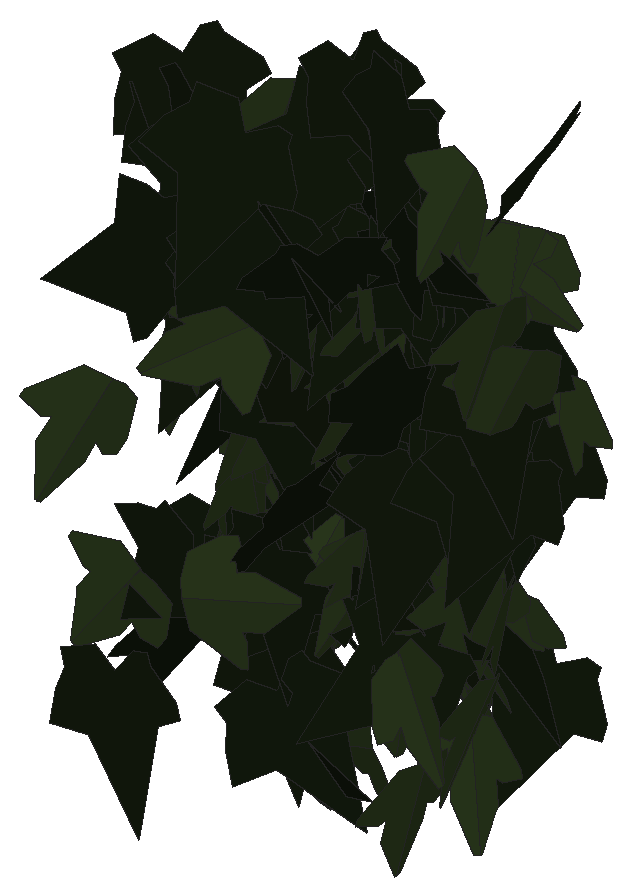
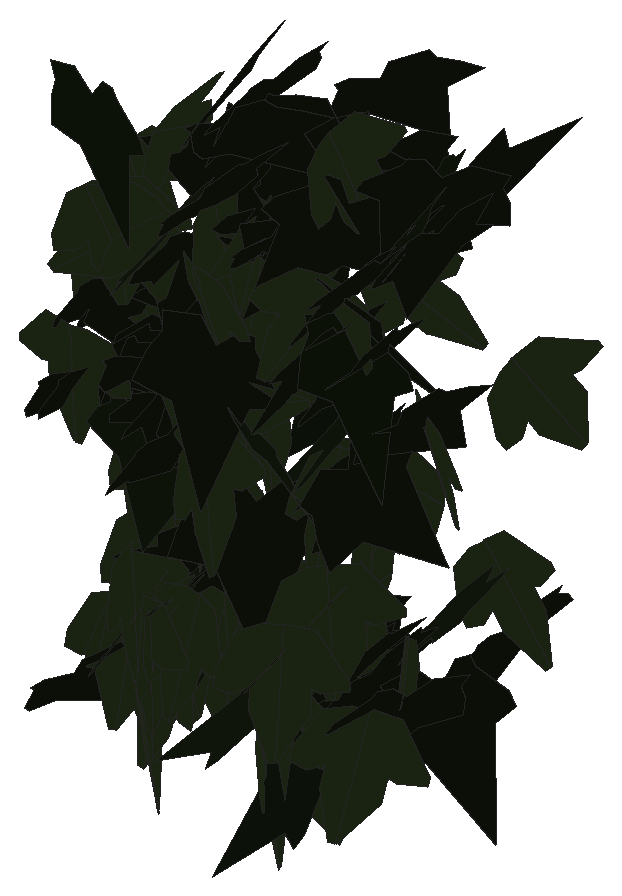
# SketchUp Ruby script. Lengths in inches.
U = 1.inch
M = Sketchup.active_model
def pt(a) = Geom::Point3d.new(a.map { |v| v * U })
def face(e, loops, mat)
  f = e.add_face(loops[0].map { |a| pt(a) })
  loops[1..].each { |l| e.add_face(l.map { |a| pt(a) }).erase! }
  f.material = f.back_material = mat if mat
  f
end
# faces: each face lists its corners as indices into pts; further lists are holes
def faces(e, pts, list, mat = nil) = list.each { |f| face(e, (f[0].is_a?(Array) ? f : [f]).map { |l| l.map { |i| pts[i] } }, mat) }
# xy, xz, yz: faces in a plane at the given z, y or x. An outline is a flat list of corners, or four numbers for a rectangle; further outlines are holes
def ring(l) = l.size == 4 ? [[l[0], l[1]], [l[2], l[1]], [l[2], l[3]], [l[0], l[3]]] : l.each_slice(2).to_a
def flat(e, list, mat, &to3) = list.each { |f| face(e, (f[0].is_a?(Array) ? f : [f]).map { |l| ring(l).map { |u, v| to3.(u, v) } }, mat) }
def xy(e, z, list, mat = nil) = flat(e, list, mat) { |x, y| [x, y, z] }
def xz(e, y, list, mat = nil) = flat(e, list, mat) { |x, z| [x, y, z] }
def yz(e, x, list, mat = nil) = flat(e, list, mat) { |y, z| [x, y, z] }
def lines(e, pts, list) = list.each { |a, b| e.add_line(pt(pts[a]), pt(pts[b])) }
# prism: a flat outline (further loops are holes) pulled along v
def prism(e, loops, v, mat = nil)
  f = face(e, loops, mat); d = Geom::Vector3d.new(v.map { |x| x * U })
  f.pushpull(f.normal.samedirection?(d) ? d.length : -d.length)
end
def box(e, o, s, mat = nil) = prism(e, [[o, [o[0] + s[0], o[1], o[2]], [o[0] + s[0], o[1] + s[1], o[2]], [o[0], o[1] + s[1], o[2]]]], [0, 0, s[2]], mat)
def at(x, y, z, deg = 0) = Geom::Transformation.translation(pt([x, y, z])) * Geom::Transformation.rotation(ORIGIN, Z_AXIS, deg.degrees)
def axes(o, x, y, z) = Geom::Transformation.new([*x, 0, *y, 0, *z, 0, *pt(o).to_a, 1])
def part(name) = M.definitions.add(name)
# library, detail: a bought-in or finely detailed component or shape, given as its bounding box
def library(name, o, s) = part(name).tap { |d| box(d.entities, o, s) }
def detail(e, o, s) = box(e.add_group.entities, o, s)
def put(e, d, t, mat = nil) = e.add_instance(d, t).tap { |i| i.material = mat if mat }
def group(e, t, mat = nil) = e.add_group.tap { |g| g.transformation = t; g.material = mat if mat }.entities
root = M.entities
M.materials.add("efeu1").color = [18, 25, 13]
M.materials.add("efeu2").color = [43, 57, 29]
c1 = part("ivyleaf_10")
p = [[0,0.5,-0.03],[-0.0625,2.02,-0.43],[-0.19,2.01,-0.46],[-0.54,1.05,-0.29],[-0.52,0.625,-0.18],[-0.83,0.76,-0.28],
  [-1.16,0.64,-0.33],[-1.15,0.33,-0.24],[-0.77,-0.39,0.02],[-0.3,-0.51,0.16],[0.04,-0.48,0.23],[-0.02,2.01,-0.4375],
  [-0.06,2.01,-0.43],[0.04,-0.49,0.23],[0.67,-0.49,0.14],[1.38,0.36,-0.2],[1.375,0.51,-0.24],[0.81,0.65,-0.19],
  [0.62,0.59,-0.15],[0.6,1.09,-0.28],[0.5,1.23,-0.31]]
faces(c1.entities,p,[[0,1,2,3,4,5,6,7,8,9,10],[11,12,0,13,14,15,16,17,18,19,20]],"efeu2")
c2 = part("ivyleaf_9")
p = [[1.54,2.16,1.25],[1.36,2.04,1.19],[-0.21,0.99,0.68],[-0.71,1.11,0.82],[-0.85,0.86,0.67],[-0.8,0.17,0.21],
  [-0.9,-0.01,0.1],[-0.67,-0.16,-0.02],[-0.08,-0.08,-0.05],[-0.03,-0.6,-0.4],[0.65,-0.88,-0.66],[0.83,-0.6,-0.49],
  [1.29,-0.42,-0.43],[1.8125,-0.07,-0.26],[1.21,0.44,0.15]]
faces(c2.entities,p,[[0,1,2,3,4,5,6,7,8,9,10,11,12,13,14]],"efeu1")
put(root,c1,axes([30.6875,222.58,242.9],[-0.44057,-0.22233,-0.08041],[0.0674,0.04488,-0.4934],[0.22661,-0.44559,-0.00958]))
put(root,c2,axes([30.85,221.21,242.7],[-0.04956,0.42875,-0.25242],[0.01989,-0.25176,-0.43153],[-0.49714,-0.05281,0.0079]))
put(root,c2,axes([30.53,222.15,243.15],[0.04788,-0.4175,-0.27092],[0.04263,0.27461,-0.41566],[0.49587,0.0167,0.06189]))
put(root,c1,axes([31.03,220.24,243.5],[-0.38302,-0.03283,0.31972],[-0.30495,-0.11998,-0.37764],[0.10152,-0.48428,0.07189]))
put(root,c1,axes([30.85,219.97,245.4],[-0.17761,-0.35591,0.30295],[-0.01741,-0.31883,-0.38477],[0.46707,-0.14722,0.10086]))
put(root,c2,axes([30.625,221.55,247.65],[0.05449,-0.47877,-0.13345],[-0.02033,0.13199,-0.48183],[0.49661,0.05793,-0.00509]))
put(root,c1,axes([30.84,221.72,243.2],[0.20355,-0.37433,-0.26162],[0.0043,0.28799,-0.40871],[0.45667,0.16414,0.12045]))
put(root,c2,axes([30.67,221.46,248.16],[-0.10102,-0.34742,-0.3451],[0.15224,0.31262,-0.35929],[0.46542,-0.17767,0.04262]))
put(root,c1,axes([30.85,221.37,245.48],[0.38535,-0.31856,0.00527],[0.00218,-0.00562,-0.49996],[0.31859,0.38534,-0.00294]))
put(root,c2,axes([30.87,221.78,245.71],[-0.19367,-0.44322,0.12668],[-0.0312,-0.12449,-0.48325],[0.45991,-0.19508,0.02057]))
put(root,c2,axes([30.96,221.17,243.27],[-0.20265,-0.2775,0.36322],[0.04048,-0.40665,-0.28809],[0.4553,-0.08736,0.18728]))
put(root,c2,axes([30.79,221.49,247.84],[0.30364,-0.39724,-0.0029],[-0.00494,-0.00013,-0.49998],[0.39722,0.30365,-0.004]))
put(root,c1,axes([31.23,222.4,244.11],[-0.37027,-0.33239,0.04918],[-0.00503,-0.06769,-0.49537],[0.33597,-0.36733,0.04678]))
put(root,c2,axes([31.12,221.36,247.33],[-0.16184,-0.44057,0.17236],[-0.03359,-0.17101,-0.46864],[0.47189,-0.16327,0.02576]))
put(root,c2,axes([31.28,221.97,245.15],[-0.13045,0.21943,-0.42992],[0.13528,-0.41088,-0.25075],[-0.46334,-0.18174,0.04783]))
put(root,c2,axes([31.39,221.81,246.35],[-0.115,0.48614,-0.02096],[0.00787,-0.01967,-0.49955],[-0.48653,-0.11522,-0.00312]))
put(root,c2,axes([31.1,219.94,242.69],[0.06343,-0.49327,-0.05162],[0.00258,0.05236,-0.49724],[0.49595,0.06282,0.00919]))
put(root,c2,axes([31.04,221.91,247.35],[0.20706,-0.40476,-0.20807],[0.02398,0.23798,-0.43908],[0.45448,0.17186,0.11797]))
put(root,c1,axes([31.4,222.88,243.65],[-0.46203,-0.18901,0.02831],[-0.02392,-0.01628,-0.49916],[0.18961,-0.46261,0.006]))
put(root,c1,axes([31.41,221.41,244.39],[0.04994,-0.46136,-0.18615],[0.0358,0.18993,-0.46113],[0.49621,0.03273,0.052]))
put(root,c2,axes([31.51,220.06,247.01],[-0.1384,-0.13116,0.46221],[-0.24658,-0.39344,-0.18548],[0.41236,-0.27929,0.04422]))
put(root,c2,axes([31.27,221.6875,242.97],[-0.01062,-0.49707,0.053],[0.00175,-0.05305,-0.49718],[0.49988,-0.01038,0.00286]))
put(root,c2,axes([31.27,221.99,246.2],[-0.00982,-0.48816,0.10773],[0.01063,-0.10793,-0.4881],[0.49979,-0.00729,0.0125]))
put(root,c1,axes([31.48,221.4,244.86],[0.08702,-0.44971,-0.20046],[0.03419,0.2086,-0.45312],[0.49118,0.06515,0.06706]))
put(root,c2,axes([31.28,222.62,242.38],[0.46432,-0.1646,-0.08553],[-0.07828,0.03514,-0.49258],[0.16817,0.47082,0.00686]))
put(root,c2,axes([31.82,221.58,246.51],[-0.47168,0.10676,0.12695],[-0.12362,0.0289,-0.48361],[-0.1106,-0.48761,-0.00087]))
put(root,c1,axes([31.45,222.46,242.97],[0.44719,-0.197,0.10591],[0.09994,-0.03582,-0.4886],[0.20009,0.45816,0.00734]))
put(root,c1,axes([31.6,222.26,242.3],[0.06401,-0.4748,0.14307],[0.00617,-0.14348,-0.47893],[0.49585,0.06308,-0.01251]))
put(root,c2,axes([31.46,221.83,242.97],[-0.06892,-0.47266,0.14778],[0.02122,-0.15189,-0.4759],[0.49477,-0.05933,0.041]))
put(root,c1,axes([31.75,221.54,248.07],[-0.0543,-0.46289,0.18107],[0.03085,-0.18494,-0.46352],[0.49608,-0.03917,0.04865]))
put(root,c1,axes([31.73,221.625,244.8],[-0.13647,-0.44588,-0.18046],[0.06991,0.16721,-0.466],[0.47591,-0.15242,0.01671]))
put(root,c2,axes([31.52,221.64,245.13],[0.13789,-0.47684,-0.06007],[-0.00645,0.06065,-0.49627],[0.48057,0.13764,0.01057]))
put(root,c2,axes([31.53,221.91,246.44],[0.21278,-0.37015,-0.26021],[-0.04577,0.26847,-0.41932],[0.45014,0.20227,0.08036]))
put(root,c1,axes([32,220.43,246.28],[0.29063,0.04582,-0.40427],[-0.40574,-0.00419,-0.29216],[-0.03016,0.49788,0.03474]))
put(root,c2,axes([31.5,222.34,243.65],[0.21833,-0.44515,-0.0646],[0.01115,0.07714,-0.49389],[0.44967,0.21422,0.04362]))
put(root,c1,axes([31.68,221.89,246.71],[-0.40611,-0.13533,-0.25838],[0.26907,-0.00287,-0.42142],[0.11258,-0.48133,0.07516]))
put(root,c2,axes([31.68,221.57,247.57],[-0.0162,-0.20911,-0.45388],[0.05645,0.45045,-0.20955],[0.49654,-0.05803,0.00901]))
put(root,c1,axes([31.73,221.55,242.83],[0.28317,0.29951,-0.28303],[0.19805,0.20225,0.41216],[0.36138,-0.34553,-0.00409]))
put(root,c2,axes([31.83,221.88,243.23],[-0.18152,-0.35458,0.3022],[-0.00969,-0.32139,-0.38291],[0.46579,-0.14487,0.10981]))
put(root,c1,axes([31.87,221.11,242.27],[0.13883,-0.33968,-0.33962],[0.08366,0.36522,-0.33109],[0.473,0.03511,0.15824]))
put(root,c2,axes([31.64,221.61,245.37],[0.31318,-0.38295,-0.07257],[-0.00433,0.08968,-0.49187],[0.38974,0.30872,0.05285]))
put(root,c1,axes([31.98,222.31,242.125],[0.17377,-0.45895,-0.09572],[-0.01824,0.09539,-0.49048],[0.46848,0.17396,0.01641]))
put(root,c2,axes([31.76,221.44,243.51],[0.06474,-0.48526,0.10162],[0.03592,-0.09763,-0.48906],[0.49449,0.07062,0.02222]))
put(root,c2,axes([31.88,221.38,242.68],[0.02552,-0.49713,-0.04705],[-0.00272,0.04697,-0.49778],[0.49934,0.02566,-0.00031]))
put(root,c2,axes([32.09,220.49,248.28],[-0.28809,-0.40854,0.00987],[-0.00353,-0.00959,-0.4999],[0.40864,-0.2881,0.00264]))
put(root,c2,axes([32.28,222.1,244.5],[0.24076,0.36214,-0.24676],[-0.1994,-0.16018,-0.42963],[-0.39022,0.30528,0.0673]))
put(root,c2,axes([31.88,222.55,242.8125],[0.34774,-0.35832,-0.02611],[0.06561,0.09906,-0.48568],[0.35323,0.33435,0.11592]))
put(root,c2,axes([32.5,222.05,245.37],[-0.39957,0.29533,0.05591],[-0.0428,0.03617,-0.49685],[-0.29751,-0.40184,-0.00362]))
put(root,c2,axes([32.61,221.24,247.93],[-0.36763,0.05194,0.33489],[-0.33529,0.0161,-0.37057],[-0.04928,-0.49703,0.023]))
put(root,c1,axes([32.35,222.13,243.38],[-0.03825,-0.35738,0.34758],[0.01463,-0.34926,-0.3575],[0.49832,-0.01718,0.03718]))
put(root,c1,axes([32.37,221.97,243.54],[-0.03084,-0.48215,0.12877],[-0.00674,-0.1286,-0.48313],[0.499,-0.03154,0.00144]))
put(root,c1,axes([32.37,222.7,245.18],[-0.02522,-0.49451,-0.06947],[-0.00212,0.06967,-0.49512],[0.49936,-0.02468,-0.00561]))
put(root,c2,axes([32.2,220.29,247.4375],[-0.01635,-0.34475,-0.36177],[0.05564,0.35846,-0.34411],[0.49663,-0.05151,0.02664]))
put(root,c1,axes([32.4375,221.32,246.5],[0.07134,-0.47542,0.13744],[0.00878,-0.13762,-0.48061],[0.49481,0.07099,-0.01129]))
put(root,c2,axes([32.38,221.7,247.1],[-0.21165,-0.41471,0.18226],[0.01095,-0.2058,-0.45555],[0.45286,-0.18885,0.0962]))
put(root,c2,axes([32.57,222.34,246.11],[0.06545,0.49561,-0.00949],[0.00783,-0.0106,-0.49983],[-0.49564,0.06528,-0.00915]))
put(root,c1,axes([32.08,220.04,243.82],[0.10382,-0.02714,-0.48835],[0.48202,-0.07899,0.10686],[-0.08295,-0.49298,0.00976]))
put(root,c1,axes([32.76,222.34,245.37],[0.09012,0.12405,0.47591],[-0.34823,-0.32557,0.1508],[0.3473,-0.35863,0.02772]))
put(root,c2,axes([32.11,221,241.94],[0.19844,-0.19315,0.41631],[0.31177,-0.27611,-0.2767],[0.33678,0.3694,0.01085]))
put(root,c1,axes([32.6,221.53,245.34],[0.06208,-0.48946,-0.08108],[0.01455,0.08348,-0.49277],[0.49592,0.05882,0.02461]))
put(root,c2,axes([32.69,221.91,248.22],[-0.38557,-0.31097,0.06803],[-0.03845,-0.06058,-0.49482],[0.316,-0.38681,0.0228]))
put(root,c1,axes([32.74,222.34,244.96],[-0.35618,0.33173,0.11442],[-0.1476,0.00628,-0.47768],[-0.31836,-0.37405,0.09345]))
put(root,c2,axes([32.54,221.79,243.44],[0.33933,-0.19776,-0.30943],[-0.22313,0.22359,-0.38758],[0.29167,0.40112,0.06349]))
put(root,c2,axes([32.45,220.6,242.68],[0.06732,-0.35273,-0.34793],[0.01817,0.35264,-0.354],[0.49511,0.03502,0.0603]))
put(root,c2,axes([32.46,221.65,248.63],[0.16313,-0.4409,-0.17029],[-0.00172,0.17959,-0.46663],[0.47264,0.15283,0.05708]))
put(root,c2,axes([32.39,220.86,247.2],[0.13896,-0.33822,0.34103],[0.1726,-0.29613,-0.36403],[0.44822,0.21889,0.03446]))
put(root,c1,axes([32.72,221.48,246.36],[0.10144,-0.41706,-0.25646],[0.02577,0.26609,-0.42253],[0.48892,0.0725,0.07548]))
put(root,c1,axes([32.74,221.91,244.41],[0.12951,-0.39075,0.2838],[0.11255,-0.26132,-0.41115],[0.46964,0.17038,0.02027]))
put(root,c2,axes([32.93,220.53,247.33],[0.10923,0.41068,-0.26345],[-0.06907,-0.25424,-0.42496],[-0.48301,0.12923,0.00119]))
put(root,c1,axes([32.84,222.38,243.27],[-0.47605,0.15237,-0.01249],[0.00564,-0.02334,-0.49942],[-0.15278,-0.47564,0.0205]))
put(root,c1,axes([33.14,221.01,242.23],[-0.20509,0.06831,0.45086],[-0.42527,0.14977,-0.21614],[-0.16458,-0.47213,-0.00333]))
put(root,c2,axes([32.89,221.5625,246.8],[-0.38536,-0.31772,-0.0235],[0.0176,0.01559,-0.49945],[0.3181,-0.38576,-0.00084]))
put(root,c1,axes([32.91,221.49,246.32],[-0.01505,-0.49191,0.08832],[-0.00815,-0.0881,-0.49211],[0.49971,-0.01625,-0.00537]))
put(root,c2,axes([32.9,219.84,244.91],[0.10724,0.38473,0.3008],[0.08255,0.28925,-0.3994],[-0.48134,0.13533,-0.00148]))
put(root,c1,axes([32.86,222.1,246.57],[0.44518,-0.22611,-0.0263],[-0.02333,0.01213,-0.49931],[0.22644,0.44579,0.00025]))
put(root,c2,axes([32.82,222.2,247.5625],[-0.15029,-0.43102,0.20405],[0.00173,-0.21444,-0.45168],[0.47688,-0.13506,0.06595]))
put(root,c1,axes([33.07,221.63,242.74],[-0.20106,-0.45753,0.01545],[-0.00673,-0.01392,-0.49976],[0.45774,-0.20118,-0.00056]))
put(root,c1,axes([32.95,221.35,246.78],[-0.10393,0.48907,-0.00259],[0.00285,-0.00205,-0.49999],[-0.48907,-0.10394,-0.00236]))
put(root,c1,axes([33.04,221.65,246.97],[0.00178,-0.49914,0.02922],[0.00965,-0.02918,-0.49905],[0.4999,0.00235,0.00952]))
put(root,c1,axes([33.06,222,244.7],[0.18843,-0.44122,-0.14077],[-0.01414,0.14642,-0.47787],[0.46292,0.18407,0.0427]))
put(root,c1,axes([33.09,221.71,244.11],[0.16062,-0.47297,-0.02226],[-0.00726,0.02104,-0.4995],[0.47344,0.16079,-0.00011]))
put(root,c1,axes([33.1875,222.125,243.07],[-0.03986,-0.49463,0.06121],[0.00431,-0.06175,-0.49615],[0.49839,-0.03903,0.00918]))
put(root,c2,axes([33.05,222.26,245.42],[-0.23116,-0.42339,-0.13156],[0.12593,0.07955,-0.4773],[0.42509,-0.2538,0.06986]))
put(root,c2,axes([33,221.7,248.32],[0.00109,-0.4249,0.26355],[0.011,-0.26347,-0.42481],[0.49988,0.00673,0.00877]))
put(root,c1,axes([33.19,222.26,242.6],[-0.46135,0.19211,-0.01596],[0.013,-0.01028,-0.49973],[-0.19233,-0.46151,0.00449]))
put(root,c2,axes([33.02,222.45,245.13],[0.05669,-0.49471,-0.04526],[-0.00923,0.0445,-0.49793],[0.49669,0.0573,-0.00408]))
put(root,c2,axes([33.01,222.21,245.61],[0.10036,-0.48111,-0.09196],[-0.01616,0.09056,-0.49146],[0.48956,0.10162,0.00263]))
put(root,c2,axes([33.1,222.08,243.33],[-0.1005,-0.47085,0.13491],[0.01056,-0.13978,-0.47995],[0.48968,-0.09362,0.03804]))
put(root,c2,axes([33.27,222.22,243.81],[-0.32347,-0.36346,0.11517],[-0.03468,-0.12236,-0.48355],[0.37969,-0.32082,0.05395]))
put(root,c2,axes([32.98,221.72,243.71],[0.31391,-0.37448,-0.10595],[-0.0316,0.11115,-0.48646],[0.38789,0.31211,0.04611]))
put(root,c1,axes([33.3,222.44,242.29],[0.22584,-0.4375,-0.08713],[-0.01932,0.08797,-0.49182],[0.44567,0.22551,0.02283]))
put(root,c1,axes([33.35,222.31,243.01],[-0.40356,-0.29358,0.03076],[0.00384,-0.05733,-0.49669],[0.29516,-0.40065,0.04853]))
put(root,c2,axes([33.14,221.8,246.83],[-0.00039,-0.4515,-0.21483],[-0.00114,0.21483,-0.45149],[0.5,0.00014,-0.0012]))
put(root,c2,axes([33.3,221.75,244.58],[-0.20418,-0.4013,0.21743],[-0.04251,-0.22044,-0.44677],[0.45443,-0.20092,0.0559]))
put(root,c2,axes([33.54,221.38,243.22],[-0.44274,-0.18,0.14691],[-0.12454,-0.08305,-0.47707],[0.19614,-0.45902,0.02871]))
put(root,c2,axes([33.35,222.25,245.72],[-0.32235,-0.38217,-0.0065],[0.02299,-0.0109,-0.49935],[0.38153,-0.32223,0.0246]))
put(root,c1,axes([33.42,222.52,243.11],[-0.49649,-0.05672,0.01668],[-0.01699,0.00175,-0.49971],[0.05662,-0.49677,-0.00366]))
put(root,c1,axes([33.36,222.48,243.625],[0.01855,-0.49754,-0.04593],[0.05165,0.04762,-0.49504],[0.49698,0.01363,0.05317]))
put(root,c2,axes([32.96,221.36,247.26],[0.23948,0.00796,-0.43885],[0.4145,0.16032,0.2291],[0.14436,-0.47353,0.07019]))
put(root,c2,axes([33.65,221.88,244.57],[0.01943,0.41167,0.28311],[-0.11494,0.27941,-0.3984],[-0.48622,-0.0496,0.10549]))
put(root,c1,axes([33.57,221.6,244.36],[-0.49857,-0.01645,0.03404],[-0.03152,-0.06773,-0.49439],[0.02088,-0.49512,0.06649]))
put(root,c2,axes([33.32,220.62,245.79],[0.15191,0.13158,0.45783],[0.33513,0.312,-0.20087],[-0.33854,0.36789,0.0066]))
put(root,c2,axes([33.48,221.25,244.86],[-0.13007,-0.4808,0.04376],[-0.00003,-0.04531,-0.49794],[0.48279,-0.12954,0.01176]))
put(root,c1,axes([33.67,221.6875,244.58],[-0.28189,-0.41093,0.0409],[-0.02571,-0.03196,-0.49832],[0.41216,-0.28304,-0.00311]))
put(root,c2,axes([33.38,222.41,243.22],[0.28335,-0.40175,-0.09115],[-0.04028,0.08309,-0.4914],[0.40999,0.28582,0.01472]))
put(root,c2,axes([33.38,222,246.9375],[0.25422,-0.42792,-0.04747],[0.01544,0.06415,-0.49563],[0.43027,0.25053,0.04583]))
put(root,c1,axes([33.71,221.75,243.59],[-0.26387,-0.42461,-0.00861],[0.00664,0.00601,-0.49992],[0.42465,-0.26394,0.00246]))
put(root,c1,axes([33.6,221.71,247.73],[-0.15621,-0.19961,0.43099],[0.21673,-0.43367,-0.1223],[0.42264,0.14861,0.22201]))
put(root,c1,axes([33.91,222.14,247.07],[-0.41024,-0.27605,0.07414],[0.00596,-0.13793,-0.48056],[0.28577,-0.39341,0.11647]))
put(root,c1,axes([33.93,220.6875,242.3],[-0.01252,-0.49822,0.04024],[0.00634,-0.0404,-0.49832],[0.4998,-0.01196,0.00733]))
put(root,c2,axes([33.84,222.72,242.52],[-0.21754,-0.44211,0.08494],[0.00745,-0.09786,-0.49027],[0.45014,-0.21204,0.04916]))
put(root,c1,axes([33.65,222.04,246.93],[-0.29636,-0.07653,-0.39537],[0.39322,0.05095,-0.30461],[0.08691,-0.49148,0.02999]))
put(root,c2,axes([34.19,222.07,248.02],[-0.18688,0.45234,0.10229],[-0.0356,0.09596,-0.48941],[-0.4624,-0.1902,-0.00366]))
put(root,c1,axes([33.82,221.53,242.29],[0.47683,-0.02754,0.1479],[0.1496,0.03478,-0.47583],[0.01592,0.49803,0.04141]))
put(root,c1,axes([34.01,221.48,242.79],[0.14159,-0.44367,0.18196],[0.04144,-0.17769,-0.46552],[0.47774,0.14691,-0.01355]))
put(root,c2,axes([33.96,221.99,246.23],[-0.06844,-0.49002,-0.07211],[0.00008,0.07279,-0.49467],[0.49529,-0.06773,-0.00988]))
put(root,c2,axes([34.02,221.55,245.11],[-0.18628,-0.45496,-0.09119],[0.0734,0.06814,-0.48987],[0.45816,-0.19589,0.0414]))
put(root,c2,axes([34.02,221.58,246.07],[0.03907,-0.48626,-0.10967],[-0.01672,0.10866,-0.48776],[0.49819,0.04178,-0.00777]))
put(root,c2,axes([34.0625,222.15,245.36],[-0.06288,-0.49603,0.00085],[-0.0094,0.00033,-0.49991],[0.49594,-0.06289,-0.00937]))
put(root,c2,axes([34.2,222.18,245.27],[-0.17293,-0.46914,0.00222],[-0.00039,-0.00223,-0.49999],[0.46914,-0.17293,0.00041]))
put(root,c1,axes([33.99,220.4,243.48],[0.32652,-0.04497,0.37598],[0.37322,-0.04562,-0.32958],[0.06395,0.49588,0.00378]))
put(root,c1,axes([34.21,222.3,245.58],[0.49838,-0.00643,0.03976],[0.04027,0.07182,-0.49317],[0.00063,0.49477,0.0721]))
put(root,c1,axes([34.41,221.54,246.27],[-0.14964,-0.43669,0.19212],[-0.05091,-0.18559,-0.46148],[0.47436,-0.15767,0.01108]))
put(root,c1,axes([34.38,221.21,246.875],[-0.03504,-0.49259,0.07825],[-0.00724,-0.07793,-0.49384],[0.49872,-0.03574,-0.00167]))
put(root,c2,axes([34.3,221.61,245.21],[-0.2147,-0.43674,0.11474],[-0.04162,-0.10737,-0.48656],[0.44964,-0.21848,0.00975]))
put(root,c1,axes([34.36,221.4,244.06],[0.23019,-0.42878,-0.11473],[-0.02415,0.11695,-0.48553],[0.4432,0.22907,0.03313]))
